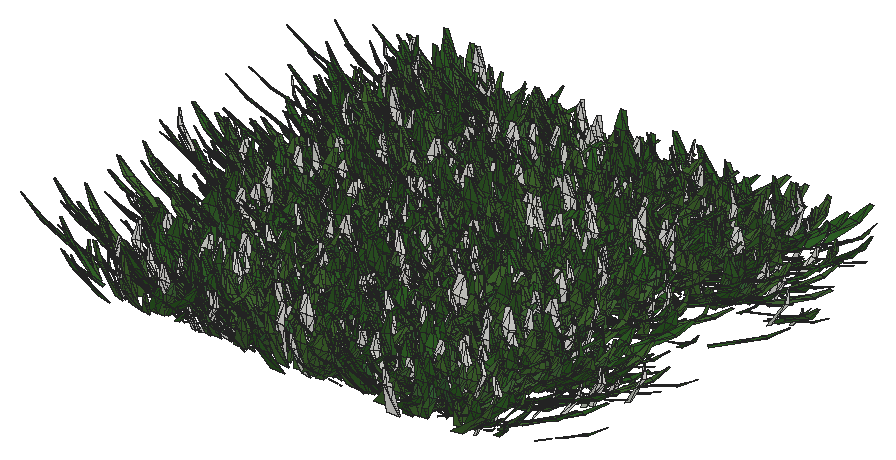
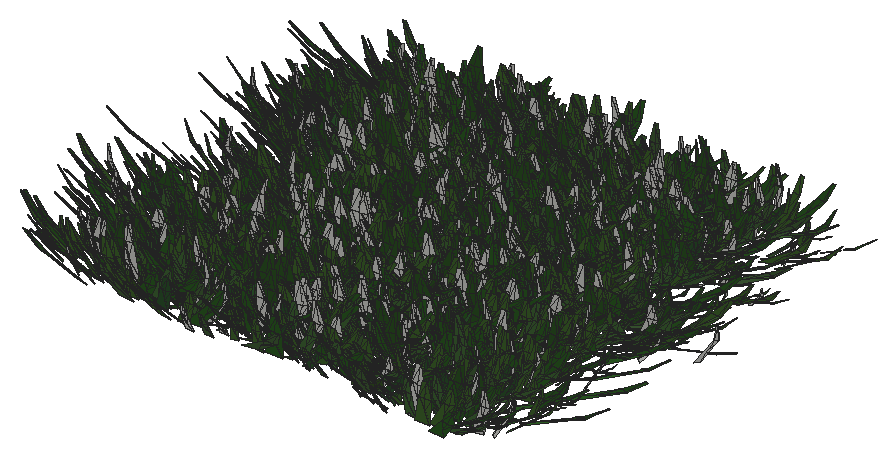
# SketchUp Ruby script. Lengths in inches.
U = 1.inch
M = Sketchup.active_model
def pt(a) = Geom::Point3d.new(a.map { |v| v * U })
def face(e, loops, mat)
  f = e.add_face(loops[0].map { |a| pt(a) })
  loops[1..].each { |l| e.add_face(l.map { |a| pt(a) }).erase! }
  f.material = f.back_material = mat if mat
  f
end
# faces: each face lists its corners as indices into pts; further lists are holes
def faces(e, pts, list, mat = nil) = list.each { |f| face(e, (f[0].is_a?(Array) ? f : [f]).map { |l| l.map { |i| pts[i] } }, mat) }
# xy, xz, yz: faces in a plane at the given z, y or x. An outline is a flat list of corners, or four numbers for a rectangle; further outlines are holes
def ring(l) = l.size == 4 ? [[l[0], l[1]], [l[2], l[1]], [l[2], l[3]], [l[0], l[3]]] : l.each_slice(2).to_a
def flat(e, list, mat, &to3) = list.each { |f| face(e, (f[0].is_a?(Array) ? f : [f]).map { |l| ring(l).map { |u, v| to3.(u, v) } }, mat) }
def xy(e, z, list, mat = nil) = flat(e, list, mat) { |x, y| [x, y, z] }
def xz(e, y, list, mat = nil) = flat(e, list, mat) { |x, z| [x, y, z] }
def yz(e, x, list, mat = nil) = flat(e, list, mat) { |y, z| [x, y, z] }
def lines(e, pts, list) = list.each { |a, b| e.add_line(pt(pts[a]), pt(pts[b])) }
# prism: a flat outline (further loops are holes) pulled along v
def prism(e, loops, v, mat = nil)
  f = face(e, loops, mat); d = Geom::Vector3d.new(v.map { |x| x * U })
  f.pushpull(f.normal.samedirection?(d) ? d.length : -d.length)
end
def box(e, o, s, mat = nil) = prism(e, [[o, [o[0] + s[0], o[1], o[2]], [o[0] + s[0], o[1] + s[1], o[2]], [o[0], o[1] + s[1], o[2]]]], [0, 0, s[2]], mat)
def at(x, y, z, deg = 0) = Geom::Transformation.translation(pt([x, y, z])) * Geom::Transformation.rotation(ORIGIN, Z_AXIS, deg.degrees)
def axes(o, x, y, z) = Geom::Transformation.new([*x, 0, *y, 0, *z, 0, *pt(o).to_a, 1])
def part(name) = M.definitions.add(name)
# library, detail: a bought-in or finely detailed component or shape, given as its bounding box
def library(name, o, s) = part(name).tap { |d| box(d.entities, o, s) }
def detail(e, o, s) = box(e.add_group.entities, o, s)
def put(e, d, t, mat = nil) = e.add_instance(d, t).tap { |i| i.material = mat if mat }
def group(e, t, mat = nil) = e.add_group.tap { |g| g.transformation = t; g.material = mat if mat }.entities
root = M.entities
M.materials.add("Material10").color = [48, 100, 38]
M.materials.add("Material3").color = [68, 110, 58]
M.materials.add("Material4").color = [48, 90, 38]
M.materials.add("Material5").color = [68, 110, 48]
M.materials.add("Material6").color = [48, 90, 48]
M.materials.add("Material7").color = [58, 110, 58]
M.materials.add("Material8").color = [58, 90, 38]
M.materials.add("Material9").color = [68, 100, 58]
c1 = part("grass00")
p = [[-0.6875,0.15,0],[-0.56,0.08,5.52],[-0.04,0.03,2.76],[0.48,-0.02,0],[0.35,-0.02,5.52],[-0.1,-0.14,5.52],
  [-0.12,0.65,8.37],[-0.42,0.65,8.37]]
faces(c1.entities,p,[[0,1,2,3],[3,2,4],[1,5,2],[5,4,2],[1,6,5],[4,5,6],[7,6,1]])
c2 = part("Group16\#1")
put(c2.entities,c1,axes([1.44,-0.61,-0.01],[0.05352,0.12609,0],[-0.10704,0.04543,0.07239],[0.06664,-0.02828,0.11628]),"Material6")
put(c2.entities,c1,axes([0.76,-0.15,-0.01],[0.04676,0.24062,0],[-0.23162,0.04501,0.06642],[0.0652,-0.01267,0.23595]),"Material3")
put(c2.entities,c1,axes([0.79,0.01,-0.01],[-0.00606,0.34651,0],[-0.34381,-0.00602,0.0432],[0.04319,0.00076,0.34386]))
put(c2.entities,c1,axes([1,0.23,-0.01],[-0.07192,0.31144,0],[-0.28722,-0.06632,0.1236],[0.12043,0.02781,0.29478]),"Material5")
put(c2.entities,c1,axes([1.66,0.77,-0.01],[-0.13828,0.29651,0],[-0.21551,-0.1005,0.22471],[0.20365,0.09498,0.23779]),"Material10")
put(c2.entities,c1,axes([0.6875,0.52,-0.01],[-0.18126,0.24051,0],[-0.22746,-0.17142,0.09788],[0.07817,0.05891,0.28481]),"Material5")
put(c2.entities,c1,axes([0.68,0.78,-0.01],[-0.215,0.18688,0],[-0.12385,-0.14248,0.21334],[0.13995,0.16101,0.18878]),"Material3")
put(c2.entities,c1,axes([0.56,1,-0.01],[-0.13756,0.07624,0],[-0.06159,-0.11112,0.0927],[0.04494,0.08108,0.12705]),"Material5")
put(c2.entities,c1,axes([0.2,0.64,-0.01],[-0.23729,0.07254,0],[-0.05711,-0.18681,0.153],[0.04473,0.14632,0.19535]),"Material10")
put(c2.entities,c1,axes([0.0625,0.72,-0.01],[-0.28874,0.02525,0],[-0.02179,-0.24916,0.14647],[0.01276,0.14591,0.25012]),"Material3")
put(c2.entities,c1,axes([-0.08,0.62,-0.01],[-0.34089,-0.04187,0],[0.03255,-0.26504,0.216],[-0.02633,0.21439,0.26703]),"Material10")
put(c2.entities,c1,axes([-0.34,0.98,-0.01],[-0.14314,-0.0493,0],[0.04397,-0.12769,0.06843],[-0.02228,0.0647,0.13505]),"Material10")
put(c2.entities,c1,axes([-0.87,1.45,-0.01],[-0.23488,-0.14114,0],[0.13761,-0.22901,0.06087],[-0.03135,0.05217,0.26717]))
put(c2.entities,c1,axes([-0.72,0.77,-0.01],[-0.14208,-0.13251,0],[0.07209,-0.0773,0.16301],[-0.11118,0.11922,0.1057]),"Material10")
put(c2.entities,c1,axes([-0.62,0.43,-0.01],[-0.14845,-0.21203,0],[0.18654,-0.13061,0.12304],[-0.10079,0.07057,0.22772]),"Material3")
put(c2.entities,c1,axes([-0.68,0.29,-0.01],[-0.13639,-0.32136,0],[0.31723,-0.13464,0.05579],[-0.05136,0.0218,0.34462]),"Material4")
put(c2.entities,c1,axes([-0.64,0.125,-0.01],[-0.0458,-0.23569,0],[0.22124,-0.043,0.08276],[-0.08124,0.01579,0.22538]),"Material7")
put(c2.entities,c1,axes([-1.6,-0.03,-0.01],[0.00576,-0.32897,0],[0.27526,0.00482,0.18018],[-0.18015,-0.00315,0.2753]),"Material5")
put(c2.entities,c1,axes([-1.36,-0.31,-0.01],[0.05718,-0.24765,0],[0.18172,0.04196,0.17267],[-0.16825,-0.03885,0.1865]),"Material10")
put(c2.entities,c1,axes([-1.54,-0.72,-0.01],[0.06537,-0.14017,0],[0.13555,0.06321,0.03939],[-0.0357,-0.01665,0.14956]))
put(c2.entities,c1,axes([-1.19,-0.9,-0.01],[0.09597,-0.12735,0],[0.11214,0.08451,0.07557],[-0.06035,-0.04548,0.14042]),"Material9")
put(c2.entities,c1,axes([-0.47,-0.54,-0.01],[0.11588,-0.10072,0],[0.0618,0.0711,0.12124],[-0.07953,-0.0915,0.0942]))
put(c2.entities,c1,axes([-0.47,-0.84,-0.01],[0.11927,-0.0661,0],[0.06603,0.11913,0.00646],[-0.00313,-0.00565,0.13621]),"Material5")
put(c2.entities,c1,axes([-0.38,-1.24,-0.01],[0.28037,-0.08571,0],[0.0618,0.20215,0.20315],[-0.05939,-0.19428,0.21139]),"Material9")
put(c2.entities,c1,axes([-0.06,-0.66,-0.01],[0.22719,-0.01987,0],[0.01247,0.14255,0.17758],[-0.01547,-0.17691,0.1431]),"Material8")
put(c2.entities,c1,axes([0.11,-0.89,-0.01],[0.14882,0.01828,0],[-0.01058,0.08611,0.12229],[0.01491,-0.12138,0.08676]),"Material6")
put(c2.entities,c1,axes([0.25,-0.72,-0.01],[0.20481,0.07053,0],[-0.06206,0.18022,0.10291],[0.03351,-0.0973,0.1906]),"Material6")
put(c2.entities,c1,axes([0.85,-1.42,-0.01],[0.16481,0.09904,0],[-0.09472,0.15762,0.05616],[0.02893,-0.04814,0.18389]),"Material5")
put(c2.entities,c1,axes([1.01,-1.09,-0.01],[0.21858,0.20385,0],[-0.17495,0.1876,0.15339],[0.10462,-0.11218,0.25652]),"Material10")
put(c2.entities,c1,axes([1.01,-0.71,-0.01],[0.08733,0.12473,0],[-0.06445,0.04512,0.13037],[0.1068,-0.07477,0.07867]),"Material6")
c3 = part("Group15\#1")
put(c3.entities,c2,at(0,0,0))
c4 = part("3darcstudiotree_grass00\#1")
put(c4.entities,c3,at(0,0,0))
put(root,c4,axes([191.21,62.81,7.6],[2.9171,1.0312,0],[-3.90665,0.69071,-0.03132],[-0.15312,0.02707,1.7905]))
put(root,c4,axes([193.61,76.57,7.6],[-3.12061,-0.47334,0],[2.372,-0.97738,-0.04577],[0.16283,-0.06709,1.96036]))
put(root,c4,axes([194.14,74.7,7.6],[-4.51264,-0.18826,0],[0.71719,-1.07444,-0.03361],[0.0313,-0.04689,1.54092]))
put(root,c4,axes([194.125,43.19,7.6],[-2.99891,-0.51884,0],[2.25803,-0.81571,-0.03348],[0.14398,-0.05201,1.87437]))
put(root,c4,axes([194.51,64.29,7.6],[-1.81184,-1.16372,0],[3.89157,-0.37868,-0.00938],[0.0544,-0.00529,1.62403]))
put(root,c4,axes([194.63,57.18,7.6],[-2.30449,-0.91323,0],[3.99186,-0.62958,-0.04882],[0.19366,-0.03054,1.38366]))
put(root,c4,axes([194.49,68.83,7.6],[-3.97113,-0.2451,0],[1.12308,-1.13729,-0.03453],[0.04096,-0.04148,1.44935]))
put(root,c4,axes([193.29,72.65,7.6],[0.9039,1.10782,0],[-3.7396,0.1907,-0.03877],[-0.30879,0.01575,1.93915]))
put(root,c4,axes([193.7,53.45,7.6],[4.31287,-0.5541,0],[2.34742,1.14195,-0.04443],[0.08836,0.04298,1.39643]))
put(root,c4,axes([195.08,59.48,7.6],[-2.23159,-0.76023,0],[4.05726,-0.74436,-0.05528],[0.25257,-0.04634,1.78248]))
put(root,c4,axes([195.1,58.8,7.6],[-4.02658,-0.46054,0],[1.58874,-0.86816,-0.02741],[0.08919,-0.04874,1.86713]))
put(root,c4,axes([193.31,61.67,7.6],[4.23303,0.24806,0],[-0.88984,0.94903,-0.007],[-0.01026,0.01094,1.56436]))
put(root,c4,axes([193.59,66.2,7.6],[0.42645,1.00239,0],[-4.44972,0.11832,-0.05804],[-0.28832,0.00767,1.39706]))
put(root,c4,axes([193.58,80.9,7.6],[3.77106,0.1861,0],[-0.77685,0.98386,-0.02055],[-0.02979,0.03773,1.87683]))
put(root,c4,axes([195.52,50.89,7.6],[-3.30832,-0.44964,0],[1.76308,-0.81076,-0.02167],[0.05991,-0.02755,1.33527]))
put(root,c4,axes([195.37,70.9,7.6],[-4.45965,0.06137,0],[-0.23794,-1.08073,-0.00024],[-0.00009,-0.00042,1.85086]))
put(root,c4,axes([195.08,45.03,7.6],[-3.86065,0.46316,0],[-1.72487,-0.89859,-0.02803],[-0.09373,-0.04883,1.92571]))
put(root,c4,axes([194.11,82.52,7.6],[0.27692,1.06146,0],[-3.97037,0.06474,-0.03468],[-0.23973,0.00391,1.72254]))
put(root,c4,axes([194.6,55.53,7.6],[4.229,-0.39119,0],[1.33455,0.9017,-0.04569],[0.11742,0.07934,1.78027]))
put(root,c4,axes([196.01,79.68,7.6],[-4.92673,0.10496,0],[-0.34343,-1.00748,-0.04489],[-0.0281,-0.08244,1.86365]))
put(root,c4,axes([195.46,52.16,7.6],[2.71553,-0.59411,0],[3.06461,0.87548,-0.0129],[0.0406,0.0116,1.39029]))
put(root,c4,axes([195.16,63.53,7.6],[4.13058,-0.51477,0],[2.24071,1.12373,-0.00236],[0.00471,0.00236,1.40454]))
put(root,c4,axes([196.47,78.61,7.6],[-4.32782,-0.07969,0],[0.34618,-1.17501,-0.00991],[0.00419,-0.01422,1.69565]))
put(root,c4,axes([195.11,47.65,7.6],[4.87575,-0.07031,0],[0.2378,1.03062,-0.03809],[0.01526,0.06615,1.79573]))
put(root,c4,axes([195.58,46.68,7.6],[4.34695,-0.61956,0],[2.03841,0.89387,-0.05304],[0.19031,0.08345,1.86337]))
put(root,c4,axes([197.13,49.18,7.6],[-0.06657,-0.97228,0],[3.61389,-0.01547,-0.01279],[0.09363,-0.0004,1.65408]))
put(root,c4,axes([197.0625,67.64,7.6],[-0.52118,1.08575,0],[-3.57431,-0.10723,-0.01529],[-0.11274,-0.00338,1.67142]))
put(root,c4,axes([199.26,49.8,7.6],[-0.33547,-0.93865,0],[4.62281,-0.10326,-0.01785],[0.11677,-0.00261,1.90542]))
put(root,c4,axes([199.35,50.34,7.6],[0.01005,-1.20258,0],[4.19815,0.00219,-0.00952],[0.05269,0.00003,1.45276]))
put(root,c4,axes([199.92,67.07,7.6],[-4.31518,-0.12187,0],[0.57213,-1.26614,-0.03054],[0.01977,-0.04376,1.83699]))
put(root,c4,axes([200.04,72.23,7.6],[-3.97014,0.26009,0],[-1.01896,-0.97211,-0.00505],[-0.00887,-0.00846,1.74136]))
put(root,c4,axes([199.29,61.38,7.6],[3.84845,-0.37536,0],[1.314,0.842,-0.03886],[0.09501,0.06088,1.52001]))
put(root,c4,axes([201.1,81.17,7.6],[-3.84586,-0.50053,0],[1.98165,-0.95164,-0.02288],[0.06035,-0.02898,1.53217]))
put(root,c4,axes([201.12,66.25,7.6],[1.58704,-0.95278,0],[3.80003,0.3956,-0.04485],[0.25602,0.02665,1.59096]))
put(root,c4,axes([200.16,47.58,7.6],[0.72703,0.98679,0],[-4.37824,0.20161,-0.0472],[-0.24448,0.01126,1.46547]))
put(root,c4,axes([200.28,63.22,7.6],[2.85718,1.03717,0],[-3.15985,0.54404,-0.04649],[-0.2079,0.0358,1.30192]))
put(root,c4,axes([200.4,55.03,7.6],[4.19495,0.19536,0],[-0.69064,0.92689,-0.03922],[-0.04451,0.05974,1.46066]))
put(root,c4,axes([201,64.99,7.6],[3.26699,-0.39523,0],[1.71248,0.88472,-0.0104],[0.02647,0.01367,1.43546]))
put(root,c4,axes([200.34,73.08,7.6],[0.48352,1.11677,0],[-5.03625,0.13628,-0.03135],[-0.15085,0.00408,1.53244]))
put(root,c4,axes([201.02,74.98,7.6],[4.15736,-0.22719,0],[0.90665,1.03692,-0.02018],[0.02441,0.02792,1.50307]))
put(root,c4,axes([203.17,58.07,7.6],[-2.6745,-0.8431,0],[3.5822,-0.71022,-0.01126],[0.04091,-0.00811,1.32461]))
put(root,c4,axes([202.8125,54.39,7.6],[-3.71389,-0.2193,0],[0.91243,-0.96576,-0.01801],[0.02228,-0.02358,1.33554]))
put(root,c4,axes([202.68,52.125,7.6],[-1.37594,-0.94184,0],[3.46555,-0.31643,-0.03784],[0.25579,-0.02336,1.65933]))
put(root,c4,axes([203.11,77.86,7.6],[-0.30959,-1.20063,0],[5.07298,-0.08176,-0.03565],[0.17141,-0.00276,1.53082]))
put(root,c4,axes([203.29,59.84,7.6],[-5.13737,-0.16678,0],[0.63051,-1.21389,-0.02421],[0.01691,-0.03256,1.66024]))
put(root,c4,axes([202.29,76.91,7.6],[2.61832,-0.717,0],[3.31257,0.75605,-0.05494],[0.2657,0.06064,1.83588]))
put(root,c4,axes([202.32,46.24,7.6],[4.35597,0.12735,0],[-0.44802,0.95775,-0.0104],[-0.00937,0.02004,1.87036]))
put(root,c4,axes([203.25,71.07,7.6],[2.88619,-0.79207,0],[3.8321,0.87272,-0.04921],[0.18723,0.04264,1.66765]))
put(root,c4,axes([203.11,69.27,7.6],[-2.47521,0.9479,0],[-4.1372,-0.67521,-0.02867],[-0.13874,-0.02264,1.78429]))
put(root,c4,axes([202.59,43.6,7.6],[3.15699,0.44702,0],[-1.9309,0.8523,-0.02459],[-0.09443,0.04168,1.90817]))
put(root,c4,axes([203.35,57.27,7.6],[4.16611,-0.6608,0],[2.43007,0.95755,-0.04672],[0.16308,0.06426,1.84728]))
put(root,c4,axes([202.68,44.36,7.6],[3.70483,0.88926,0],[-3.42802,0.89261,-0.04664],[-0.18584,0.04839,1.77978]))
put(root,c4,axes([203.33,79.36,7.6],[1.28426,1.18436,0],[-4.11752,0.27905,-0.02312],[-0.12583,0.00853,1.50331]))
put(root,c4,axes([205.93,59.6,7.6],[2.28346,-0.77469,0],[3.44717,0.63505,-0.04551],[0.22499,0.04145,1.64335]))
put(root,c4,axes([205.96,55.37,7.6],[-3.11661,0.81451,0],[-3.35485,-0.80231,-0.01205],[-0.05625,-0.01345,1.87482]))
put(root,c4,axes([207.1,48.41,7.6],[-4.56857,-0.03056,0],[0.12408,-1.1593,-0.01377],[0.0021,-0.01961,1.65227]))
put(root,c4,axes([206.63,65.01,7.6],[-3.49798,0.58152,0],[-2.29705,-0.86358,-0.00165],[-0.005,-0.00188,1.42237]))
put(root,c4,axes([207.66,52.14,7.6],[-3.54461,-0.42652,0],[2.22844,-1.15748,-0.00367],[0.00795,-0.00413,1.60507]))
put(root,c4,axes([207.23,46.23,7.6],[0.72449,-1.28293,0],[4.25597,0.15021,-0.01886],[0.1212,0.00428,1.74385]))
put(root,c4,axes([206.16,62.66,7.6],[4.06118,0.1391,0],[-0.5324,0.97148,-0.00884],[-0.00926,0.01689,1.89082]))
put(root,c4,axes([206.31,80.17,7.6],[3.80962,0.48399,0],[-2.27163,1.11755,-0.02666],[-0.05719,0.02813,1.48409]))
put(root,c4,axes([206.93,44.37,7.6],[-1.84818,0.79503,0],[-4.49204,-0.65265,-0.02835],[-0.13063,-0.01898,1.73088]))
put(root,c4,axes([208.52,75.28,7.6],[-4.49893,-0.43837,0],[1.53995,-0.98776,-0.03755],[0.08017,-0.05142,1.55797]))
put(root,c4,axes([206.94,73.21,7.6],[4.7752,0.14497,0],[-0.46713,0.96169,-0.01966],[-0.01749,0.036,1.78732]))
put(root,c4,axes([207.42,67.24,7.6],[-1.92575,0.83965,0],[-4.05155,-0.58077,-0.01882],[-0.10891,-0.01561,1.94745]))
put(root,c4,axes([209.1,72.56,7.6],[-1.58063,-0.88051,0],[4.29272,-0.48163,-0.01184],[0.05795,-0.0065,1.57815]))
put(root,c4,axes([208.85,76.55,7.6],[-0.4942,-0.9258,0],[4.62783,-0.1544,-0.03174],[0.19168,-0.0064,1.77768]))
put(root,c4,axes([207.8,50.73,7.6],[4.19202,-0.62373,0],[2.32182,0.97529,-0.02674],[0.0725,0.03045,1.50406]))
put(root,c4,axes([208.98,78.26,7.6],[-2.7199,-1.09643,0],[3.70626,-0.57463,-0.05324],[0.3066,-0.04754,1.84703]))
put(root,c4,axes([208.85,61.11,7.6],[-4.05366,0.12739,0],[-0.60907,-1.21134,-0.04842],[-0.03855,-0.07666,1.94818]))
put(root,c4,axes([209.44,43.39,7.6],[-2.21429,-1.09214,0],[3.31642,-0.42025,-0.03791],[0.27447,-0.03478,1.88609]))
put(root,c4,axes([207.97,58.8125,7.6],[5.04215,0.13014,0],[-0.5216,1.26309,-0.06196],[-0.03085,0.07472,1.53928]))
put(root,c4,axes([208.21,49.05,7.6],[4.01222,0.17516,0],[-0.82819,1.18564,-0.04039],[-0.03228,0.04621,1.39779]))
put(root,c4,axes([208.48,57.29,7.6],[3.70391,0.67264,0],[-2.69019,0.92586,-0.05492],[-0.18493,0.06364,1.63919]))
put(root,c4,axes([209.78,80.78,7.6],[-3.854,0.71401,0],[-2.71385,-0.91553,-0.03727],[-0.14645,-0.04941,1.88005]))
put(root,c4,axes([209.18,66.58,7.6],[3.9405,-0.83524,0],[2.79845,0.82516,-0.04452],[0.20818,0.06139,1.95574]))
put(root,c4,axes([208.3125,69.5,7.6],[2.7963,0.73348,0],[-3.70563,0.88296,-0.0237],[-0.07242,0.01726,1.35093]))
put(root,c4,axes([209.46,54.33,7.6],[3.48051,0.83109,0],[-2.69675,0.70586,-0.00574],[-0.02303,0.00603,1.41814]))
put(root,c4,axes([209.68,70.89,7.6],[1.55604,0.87534,0],[-4.29389,0.47706,-0.00487],[-0.02529,0.00281,1.66894]))
put(root,c4,axes([212.61,46.31,7.6],[-4.60072,-0.1914,0],[0.66397,-0.99747,-0.03971],[0.03807,-0.05719,1.4765]))
put(root,c4,axes([211.88,78.39,7.6],[-2.80563,0.59342,0],[-3.19145,-0.94305,-0.04396],[-0.1676,-0.04953,1.82298]))
put(root,c4,axes([211.96,79.14,7.6],[-3.36424,0.91814,0],[-3.26593,-0.74794,-0.02313],[-0.11922,-0.0273,1.93523]))
put(root,c4,axes([211.95,50.98,7.6],[3.31986,-0.90832,0],[2.95695,0.67547,-0.04297],[0.18756,0.04285,1.48019]))
put(root,c4,axes([211.85,52.81,7.6],[4.45796,-0.3025,0],[1.23547,1.13796,-0.0215],[0.03263,0.03006,1.70776]))
put(root,c4,axes([211.59,70.41,7.6],[1.59432,0.97436,0],[-4.70635,0.4813,-0.06498],[-0.3656,0.03739,1.93183]))
put(root,c4,axes([212.21,60.37,7.6],[4.36905,-0.5157,0],[1.63569,0.86611,-0.01833],[0.04371,0.02315,1.33779]))
put(root,c4,axes([212.125,61.79,7.6],[-2.09066,0.8963,0],[-4.13643,-0.60302,-0.00159],[-0.00743,-0.00108,1.61385]))
put(root,c4,axes([212.04,74.87,7.6],[3.77784,0.09096,0],[-0.38847,1.00844,-0.03978],[-0.02973,0.07718,1.9745]))
put(root,c4,axes([212.74,67.21,7.6],[4.39293,-0.39638,0],[1.51129,1.04681,-0.00463],[0.01009,0.00699,1.7876]))
put(root,c4,axes([214.38,45.31,7.6],[-2.80912,-0.5814,0],[2.98833,-0.9024,-0.02106],[0.0666,-0.02011,1.45262]))
put(root,c4,axes([212.17,57.96,7.6],[1.32804,0.89243,0],[-4.56048,0.42416,-0.01219],[-0.04894,0.00455,1.30286]))
put(root,c4,axes([213.53,53.57,7.6],[-3.32952,0.73934,0],[-2.566,-0.72222,-0.02123],[-0.07998,-0.02251,1.37003]))
put(root,c4,axes([213.76,57.51,7.6],[1.3987,-1.16529,0],[3.94932,0.29627,-0.0465],[0.25173,0.01888,1.45674]))
put(root,c4,axes([212.75,49.08,7.6],[4.48384,-0.0442,0],[0.16896,1.07134,-0.03451],[0.00949,0.06019,1.8714]))
put(root,c4,axes([214.68,81.43,7.6],[-2.9743,-0.97046,0],[3.84774,-0.73704,-0.04805],[0.20355,-0.03899,1.61679]))
put(root,c4,axes([212.6875,47.71,7.6],[3.76585,0.33599,0],[-1.61193,1.12919,-0.03925],[-0.05722,0.04008,1.29995]))
put(root,c4,axes([214.2,76.13,7.6],[1.03504,-1.15768,0],[4.4608,0.24927,-0.0396],[0.20091,0.01123,1.48525]))
put(root,c4,axes([213.7,69.38,7.6],[3.13436,-0.48515,0],[2.36256,0.95397,-0.03178],[0.09873,0.03987,1.65559]))
put(root,c4,axes([213.39,73.24,7.6],[2.27275,0.69978,0],[-3.25332,0.66039,-0.04172],[-0.2207,0.0448,1.78477]))
put(root,c4,axes([215.07,71.84,7.6],[0.03995,-0.91638,0],[3.85114,0.01049,-0.01263],[0.08929,0.00024,1.70174]))
put(root,c4,axes([215.32,55.18,7.6],[-0.0743,-1.09346,0],[5.15443,-0.02189,-0.0635],[0.38021,-0.00161,1.92948]))
put(root,c4,axes([214.93,64.76,7.6],[-0.87822,1.20362,0],[-5.10038,-0.23259,-0.02378],[-0.14141,-0.00645,1.95907]))
put(root,c4,axes([215.26,43.59,7.6],[-1.6227,0.88053,0],[-4.355,-0.50161,-0.00587],[-0.0262,-0.00302,1.47291]))
put(root,c4,axes([215.3,65.56,7.6],[4.89448,0.02106,0],[-0.07768,1.1284,-0.04862],[-0.00413,0.05993,1.39123]))
put(root,c4,axes([215.82,62.85,7.6],[3.93844,-0.46233,0],[1.56764,0.83463,-0.03796],[0.10707,0.05701,1.52986]))
put(root,c4,axes([217.94,50.93,7.6],[-4.19523,0.01101,0],[-0.04384,-1.04387,-0.01485],[-0.00097,-0.02314,1.62647]))
put(root,c4,axes([217.83,70.87,7.6],[2.74476,-0.63144,0],[3.24378,0.88126,-0.00074],[0.00283,0.00077,1.68668]))
put(root,c4,axes([218.5,60.47,7.6],[-1.38491,-0.87134,0],[4.17889,-0.41512,-0.04918],[0.21859,-0.02171,1.34418]))
put(root,c4,axes([217.875,66.05,7.6],[-2.83927,0.94701,0],[-3.75848,-0.70428,-0.01976],[-0.09358,-0.01754,1.7373]))
put(root,c4,axes([217.61,67.47,7.6],[4.64321,-0.10228,0],[0.43492,1.23399,-0.00682],[0.00288,0.00819,1.49182]))
put(root,c4,axes([218.98,61.8,7.6],[0.60172,-0.90687,0],[4.84176,0.20079,-0.06063],[0.30013,0.01245,1.53907]))
put(root,c4,axes([217.73,76.77,7.6],[4.59228,0.4506,0],[-1.57539,1.00348,-0.00074],[-0.00157,0.001,1.56313]))
put(root,c4,axes([219.88,68.83,7.6],[-4.3908,-0.21331,0],[0.95341,-1.22655,-0.00093],[0.00081,-0.00104,1.42207]))
put(root,c4,axes([220.03,74.84,7.6],[-2.23417,-0.72587,0],[3.44566,-0.66284,-0.03027],[0.1304,-0.02509,1.47708]))
put(root,c4,axes([218.11,64.73,7.6],[0.72512,1.17526,0],[-3.95245,0.15241,-0.0058],[-0.04155,0.0016,1.813]))
put(root,c4,axes([219.48,43.18,7.6],[-3.45708,0.57656,0],[-2.12905,-0.79787,-0.03251],[-0.13485,-0.05053,1.79208]))
put(root,c4,axes([219.74,53.53,7.6],[1.59637,-0.98272,0],[4.08137,0.41437,-0.04502],[0.2819,0.02862,1.86083]))
put(root,c4,axes([219.38,46.87,7.6],[3.44919,-0.8389,0],[2.51647,0.64667,-0.01443],[0.08324,0.02139,1.86565]))
put(root,c4,axes([220.65,56.54,7.6],[-4.3854,-0.36655,0],[1.15878,-0.86648,-0.00172],[0.00341,-0.00255,1.42531]))
put(root,c4,axes([220.76,47.43,7.6],[-1.10015,-1.07569,0],[4.31851,-0.27604,-0.04783],[0.26751,-0.0171,1.6084]))
put(root,c4,axes([221.11,73.42,7.6],[-2.44496,-0.90858,0],[3.92777,-0.66059,-0.0439],[0.19033,-0.03201,1.54604]))
put(root,c4,axes([219.12,63.44,7.6],[3.01882,0.54467,0],[-2.85178,0.98787,-0.01696],[-0.0599,0.02075,1.8379]))
put(root,c4,axes([219.36,55.93,7.6],[1.72651,0.80182,0],[-4.15188,0.55875,-0.00648],[-0.03257,0.00438,1.68262]))
put(root,c4,axes([221.34,81.41,7.6],[-4.67562,0.03677,0],[-0.12525,-0.99545,-0.03177],[-0.00796,-0.06328,1.98473]))
put(root,c4,axes([219.58,77.84,7.6],[3.74443,0.79231,0],[-2.92784,0.86481,-0.04954],[-0.20172,0.05958,1.78537]))
put(root,c4,axes([221.87,48.81,7.6],[-0.41267,-0.99142,0],[5.06334,-0.13172,-0.00351],[0.0163,-0.00042,1.48465]))
put(root,c4,axes([219.91,45.38,7.6],[4.97186,0.0872,0],[-0.33381,1.18949,-0.05051],[-0.02266,0.08074,1.91076]))
put(root,c4,axes([221.88,79.86,7.6],[-2.51888,-0.8121,0],[2.88545,-0.55936,-0.0081],[0.05261,-0.0102,1.87526]))
put(root,c4,axes([221.48,72.06,7.6],[0.49939,-1.21812,0],[4.94049,0.12659,-0.06373],[0.30684,0.00786,1.50237]))
put(root,c4,axes([221.44,51.85,7.6],[1.78182,-0.82345,0],[4.25701,0.57572,-0.03985],[0.17401,0.02353,1.5017]))
put(root,c4,axes([220.96,58.29,7.6],[4.57283,0.48925,0],[-2.0405,1.19199,-0.06274],[-0.14636,0.0855,1.92197]))
put(root,c4,axes([223.59,52.94,7.6],[-4.16521,-0.5533,0],[2.06422,-0.97121,-0.03648],[0.11162,-0.05251,1.79293]))
put(root,c4,axes([223.52,51.34,7.6],[-2.37661,-1.01523,0],[3.11528,-0.4558,-0.0221],[0.1541,-0.02255,1.82262]))
put(root,c4,axes([223.5625,44.88,7.6],[3.5158,-0.29291,0],[1.43894,1.07947,-0.01535],[0.02658,0.01994,1.5577]))
put(root,c4,axes([224.98,73.94,7.6],[-3.60429,-0.54918,0],[1.97169,-0.80877,-0.03312],[0.12446,-0.05105,1.70984]))
put(root,c4,axes([224.63,76.46,7.6],[1.08767,-1.10089,0],[4.34215,0.26813,-0.04714],[0.21998,0.01358,1.34372]))
put(root,c4,axes([225.24,54.42,7.6],[-2.39381,-0.81809,0],[3.41436,-0.62442,-0.02018],[0.11154,-0.0204,1.81061]))
put(root,c4,axes([223.8,64.17,7.6],[4.48845,-0.0996,0],[0.40703,1.14637,-0.01913],[0.01094,0.03082,1.86132]))
put(root,c4,axes([225.66,70.88,7.6],[-2.33649,-0.74426,0],[3.77896,-0.74146,-0.04646],[0.22132,-0.04342,1.81816]))
put(root,c4,axes([223.66,80.6875,7.6],[3.85435,0.70628,0],[-2.80826,0.95783,-0.04132],[-0.15487,0.05282,1.88254]))
put(root,c4,axes([224.47,55.68,7.6],[-1.94964,1.12405,0],[-4.22902,-0.45845,-0.00354],[-0.01854,-0.00201,1.64409]))
put(root,c4,axes([224.1875,79.85,7.6],[3.1818,0.67229,0],[-2.74348,0.81152,-0.00305],[-0.01175,0.00348,1.58836]))
put(root,c4,axes([226.29,71.89,7.6],[-4.23791,0.69969,0],[-2.41225,-0.91316,-0.01955],[-0.05785,-0.0219,1.46911]))
